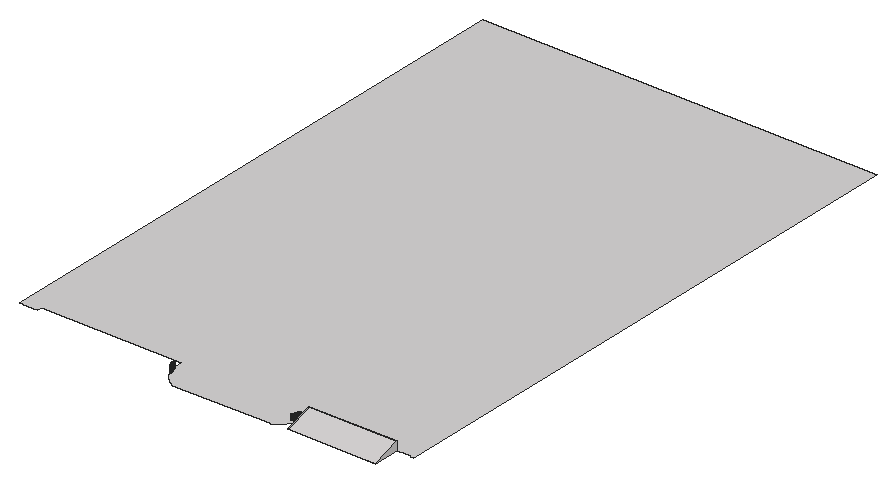
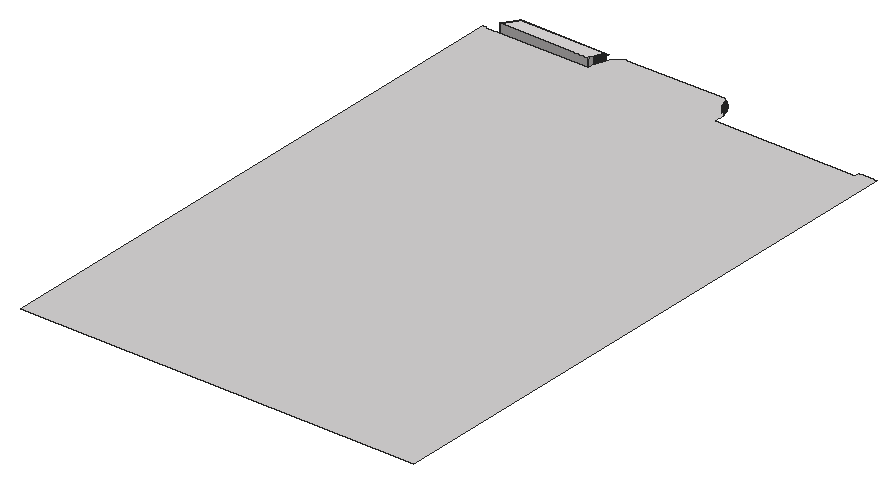
# SketchUp Ruby script. Lengths in inches.
U = 1.inch
M = Sketchup.active_model
def pt(a) = Geom::Point3d.new(a.map { |v| v * U })
def face(e, loops, mat)
  f = e.add_face(loops[0].map { |a| pt(a) })
  loops[1..].each { |l| e.add_face(l.map { |a| pt(a) }).erase! }
  f.material = f.back_material = mat if mat
  f
end
# faces: each face lists its corners as indices into pts; further lists are holes
def faces(e, pts, list, mat = nil) = list.each { |f| face(e, (f[0].is_a?(Array) ? f : [f]).map { |l| l.map { |i| pts[i] } }, mat) }
# xy, xz, yz: faces in a plane at the given z, y or x. An outline is a flat list of corners, or four numbers for a rectangle; further outlines are holes
def ring(l) = l.size == 4 ? [[l[0], l[1]], [l[2], l[1]], [l[2], l[3]], [l[0], l[3]]] : l.each_slice(2).to_a
def flat(e, list, mat, &to3) = list.each { |f| face(e, (f[0].is_a?(Array) ? f : [f]).map { |l| ring(l).map { |u, v| to3.(u, v) } }, mat) }
def xy(e, z, list, mat = nil) = flat(e, list, mat) { |x, y| [x, y, z] }
def xz(e, y, list, mat = nil) = flat(e, list, mat) { |x, z| [x, y, z] }
def yz(e, x, list, mat = nil) = flat(e, list, mat) { |y, z| [x, y, z] }
def lines(e, pts, list) = list.each { |a, b| e.add_line(pt(pts[a]), pt(pts[b])) }
# prism: a flat outline (further loops are holes) pulled along v
def prism(e, loops, v, mat = nil)
  f = face(e, loops, mat); d = Geom::Vector3d.new(v.map { |x| x * U })
  f.pushpull(f.normal.samedirection?(d) ? d.length : -d.length)
end
def box(e, o, s, mat = nil) = prism(e, [[o, [o[0] + s[0], o[1], o[2]], [o[0] + s[0], o[1] + s[1], o[2]], [o[0], o[1] + s[1], o[2]]]], [0, 0, s[2]], mat)
def at(x, y, z, deg = 0) = Geom::Transformation.translation(pt([x, y, z])) * Geom::Transformation.rotation(ORIGIN, Z_AXIS, deg.degrees)
def axes(o, x, y, z) = Geom::Transformation.new([*x, 0, *y, 0, *z, 0, *pt(o).to_a, 1])
def part(name) = M.definitions.add(name)
# library, detail: a bought-in or finely detailed component or shape, given as its bounding box
def library(name, o, s) = part(name).tap { |d| box(d.entities, o, s) }
def detail(e, o, s) = box(e.add_group.entities, o, s)
def put(e, d, t, mat = nil) = e.add_instance(d, t).tap { |i| i.material = mat if mat }
def group(e, t, mat = nil) = e.add_group.tap { |g| g.transformation = t; g.material = mat if mat }.entities
root = M.entities
M.materials.add("[Quartz Light Brown]").color = [215, 212, 212]
M.materials.add("[Stone Sandstone Ashlar Light]").color = [201, 199, 196]
xy(root,-12,[[240,0,239.65,0.16,239.29,0.32,238.59,0.66,238.25,0.83,237.9,1.01,237.56,1.19,237.21,1.375,236.53,1.75,236.2,1.95,235.86,2.14,235.2,2.54,234.21,3.17,232.93,4.05,232.62,4.28,232.3,4.51,231.99,4.74,231.6875,4.98,231.38,5.22,231.08,5.46,230.18,6.21,229.89,6.46,229.59,6.72,229.31,6.98,229.02,7.24,228.73,7.51,228.45,7.77,227.9,8.32,227.625,8.59,227.35,8.87,227.08,9.15,226.82,9.4375,226.56,9.72,226.04,10.3,225.78,10.6,225.53,10.89,225.28,11.19,225.04,11.49,224.79,11.79,224.55,12.1,224.32,12.41,224.08,12.72,223.62,13.34,223.4,13.66,223.17,13.98,222.95,14.3,222.53,14.95,222.32,15.28,222.11,15.6,221.91,15.9375,221.7,16.27,221.51,16.6,221.3125,16.94,221.12,17.28,220.94,17.62,220.75,17.96,220.57,18.31,220.39,18.65,219.88,19.7,219.72,20.05,219.55,20.4,219.4,20.76,219.24,21.12,219.09,21.47,218.95,21.83,218.8,22.2,218.52,22.92,218.39,23.29,218.26,23.65,218.14,24.02,218.01,24.39,217.89,24.76,217.67,25.5,217.45,26.25,217.25,27,217.07,27.76,216.98,28.13,216.82,28.89,216.74,29.28,216.6,30.04,216.54,30.42,216.48,30.81,216.42,31.19,216.36,31.58,216.31,31.96,216.27,32.35,216.23,32.73,216.1875,33.12,216.15,33.51,216.12,33.89,216.09,34.28,216.03,35.45,216.02,35.83,216,36.61,216,44,24,44,24,38,20,38,20,39,19,39,19,38,5,38,5,39,4,39,4,38,0,38,0,830,540,830,540,38,536,38,536,39,535,39,535,38,521,38,521,39,520,39,520,38,396,38,396,36,395.99,36,395.98,35.83,395.97,35.45,395.91,34.28,395.88,33.89,395.85,33.51,395.8125,33.12,395.77,32.73,395.73,32.35,395.69,31.96,395.64,31.58,395.58,31.19,395.52,30.81,395.46,30.42,395.4,30.04,395.26,29.28,395.18,28.89,395.02,28.13,394.93,27.76,394.75,27,394.55,26.25,394.33,25.5,394.11,24.76,393.99,24.39,393.86,24.02,393.74,23.65,393.61,23.29,393.48,22.92,393.2,22.2,393.05,21.83,392.91,21.47,392.76,21.12,392.6,20.76,392.45,20.4,392.28,20.05,392.12,19.7,391.61,18.65,391.43,18.31,391.25,17.96,391.06,17.62,390.88,17.28,390.6875,16.94,390.49,16.6,390.3,16.27,390.09,15.9375,389.89,15.6,389.68,15.28,389.47,14.95,389.05,14.3,388.83,13.98,388.6,13.66,388.38,13.34,387.92,12.72,387.68,12.41,387.45,12.1,387.21,11.79,386.96,11.49,386.72,11.19,386.47,10.89,386.22,10.6,385.96,10.3,385.44,9.72,385.18,9.4375,384.92,9.15,384.65,8.87,384.375,8.59,384.1,8.32,383.55,7.77,383.27,7.51,382.98,7.24,382.69,6.98,382.41,6.72,382.11,6.46,381.82,6.21,380.92,5.46,380.62,5.22,380.3125,4.98,380.01,4.74,379.7,4.51,379.38,4.28,379.07,4.05,377.79,3.17,376.8,2.54,376.14,2.14,375.8,1.95,375.47,1.75,374.79,1.375,374.44,1.19,374.1,1.01,373.75,0.83,373.41,0.66,372.71,0.32,372.35,0.16,372,0]],"[Quartz Light Brown]")
p = [[221.12,17.28,-3],[220.94,17.62,-3],[220.94,17.62,-12],[221.12,17.28,-12],[391.06,17.62,-3],[390.88,17.28,-3],
  [390.88,17.28,-12],[391.06,17.62,-12],[220.75,17.96,-3],[220.75,17.96,-12],[391.25,17.96,-3],[391.25,17.96,-12],
  [220.57,18.31,-3],[220.57,18.31,-12],[391.43,18.31,-3],[391.43,18.31,-12],[220.39,18.65,-3],[220.39,18.65,-12],
  [391.61,18.65,-3],[391.61,18.65,-12],[220.22,19,-3],[220.22,19,-12],[391.78,19,-3],[391.78,19,-12],
  [220.05,19.35,-3],[220.05,19.35,-12],[391.95,19.35,-3],[391.95,19.35,-12],[219.88,19.7,-3],[219.88,19.7,-12],
  [392.12,19.7,-3],[392.12,19.7,-12],[219.72,20.05,-3],[219.72,20.05,-12],[392.28,20.05,-3],[392.28,20.05,-12],
  [219.55,20.4,-3],[219.55,20.4,-12],[392.45,20.4,-3],[392.45,20.4,-12],[219.4,20.76,-3],[219.4,20.76,-12],
  [392.6,20.76,-3],[392.6,20.76,-12],[219.24,21.12,-3],[219.24,21.12,-12],[392.76,21.12,-3],[392.76,21.12,-12],
  [219.09,21.47,-3],[219.09,21.47,-12],[392.91,21.47,-3],[392.91,21.47,-12],[218.95,21.83,-3],[218.95,21.83,-12],
  [393.05,21.83,-3],[393.05,21.83,-12],[218.8,22.2,-3],[218.8,22.2,-12],[393.2,22.2,-3],[393.2,22.2,-12],
  [218.66,22.56,-3],[218.66,22.56,-12],[393.34,22.56,-3],[393.34,22.56,-12],[218.52,22.92,-3],[218.52,22.92,-12],
  [393.48,22.92,-3],[393.48,22.92,-12],[218.39,23.29,-3],[218.39,23.29,-12],[393.61,23.29,-3],[393.61,23.29,-12],
  [218.26,23.65,-3],[218.26,23.65,-12],[393.74,23.65,-3],[393.74,23.65,-12],[218.14,24.02,-3],[218.14,24.02,-12],
  [393.86,24.02,-3],[393.86,24.02,-12],[218.01,24.39,-3],[218.01,24.39,-12],[393.99,24.39,-3],[393.99,24.39,-12],
  [217.89,24.76,-3],[217.89,24.76,-12],[394.11,24.76,-3],[394.11,24.76,-12],[217.78,25.13,-3],[217.78,25.13,-12],
  [394.22,25.13,-3],[394.22,25.13,-12],[217.67,25.5,-3],[217.67,25.5,-12],[394.33,25.5,-3],[394.33,25.5,-12],
  [217.56,25.875,-3],[217.56,25.875,-12],[394.44,25.875,-3],[394.44,25.875,-12],[217.45,26.25,-3],[217.45,26.25,-12],
  [394.55,26.25,-3],[394.55,26.25,-12],[217.35,26.625,-3],[217.35,26.625,-12],[394.65,26.625,-3],[394.65,26.625,-12],
  [217.25,27,-3],[217.25,27,-12],[394.75,27,-3],[394.75,27,-12],[217.16,27.38,-3],[217.16,27.38,-12],
  [394.84,27.38,-3],[394.84,27.38,-12],[217.07,27.76,-3],[217.07,27.76,-12],[394.93,27.76,-3],[394.93,27.76,-12],
  [216.98,28.13,-3],[216.98,28.13,-12],[395.02,28.13,-3],[395.02,28.13,-12],[224.47,17.5,-3],[224.66,17.1875,-3],
  [224.66,17.1875,-10],[224.47,17.5,-10],[387.34,17.1875,-3],[387.53,17.5,-3],[387.53,17.5,-10],[387.34,17.1875,-10],
  [224.28,17.8,-3],[224.28,17.8,-10],[387.72,17.8,-3],[387.72,17.8,-10],[224.1,18.11,-3],[224.1,18.11,-10],
  [387.9,18.11,-3],[387.9,18.11,-10],[223.92,18.43,-3],[223.92,18.43,-10],[388.08,18.43,-3],[388.08,18.43,-10],
  [223.74,18.74,-3],[223.74,18.74,-10],[388.26,18.74,-3],[388.26,18.74,-10],[223.57,19.05,-3],[223.57,19.05,-10],
  [388.43,19.05,-3],[388.43,19.05,-10],[223.4,19.37,-3],[223.4,19.37,-10],[388.6,19.37,-3],[388.6,19.37,-10],
  [223.23,19.69,-3],[223.23,19.69,-10],[388.77,19.69,-3],[388.77,19.69,-10],[223.07,20.01,-3],[223.07,20.01,-10],
  [388.93,20.01,-3],[388.93,20.01,-10],[222.91,20.33,-3],[222.91,20.33,-10],[389.09,20.33,-3],[389.09,20.33,-10],
  [222.75,20.65,-3],[222.75,20.65,-10],[389.25,20.65,-3],[389.25,20.65,-10],[222.59,20.98,-3],[222.59,20.98,-10],
  [389.41,20.98,-3],[389.41,20.98,-10],[222.44,21.31,-3],[222.44,21.31,-10],[389.56,21.31,-3],[389.56,21.31,-10],
  [222.29,21.63,-3],[222.29,21.63,-10],[389.71,21.63,-3],[389.71,21.63,-10],[222.15,21.96,-3],[222.15,21.96,-10],
  [389.85,21.96,-3],[389.85,21.96,-10],[222,22.29,-3],[222,22.29,-10],[390,22.29,-3],[390,22.29,-10],
  [221.86,22.625,-3],[221.86,22.625,-10],[390.14,22.625,-3],[390.14,22.625,-10],[221.73,22.96,-3],[221.73,22.96,-10],
  [390.27,22.96,-3],[390.27,22.96,-10],[221.59,23.29,-3],[221.59,23.29,-10],[390.41,23.29,-3],[390.41,23.29,-10],
  [221.46,23.625,-3],[221.46,23.625,-10],[390.54,23.625,-3],[390.54,23.625,-10],[221.34,23.96,-3],[221.34,23.96,-10],
  [390.66,23.96,-3],[390.66,23.96,-10],[221.21,24.3,-3],[221.21,24.3,-10],[390.79,24.3,-3],[390.79,24.3,-10],
  [221.09,24.64,-3],[221.09,24.64,-10],[390.91,24.64,-3],[390.91,24.64,-10],[220.98,24.98,-3],[220.98,24.98,-10],
  [391.02,24.98,-3],[391.02,24.98,-10],[220.86,25.32,-3],[220.86,25.32,-10],[391.14,25.32,-3],[391.14,25.32,-10],
  [220.75,25.67,-3],[220.75,25.67,-10],[391.25,25.67,-3],[391.25,25.67,-10],[220.65,26.01,-3],[220.65,26.01,-10],
  [391.35,26.01,-3],[391.35,26.01,-10],[220.54,26.35,-3],[220.54,26.35,-10],[391.46,26.35,-3],[391.46,26.35,-10],
  [220.44,26.7,-3],[220.44,26.7,-10],[391.56,26.7,-3],[391.56,26.7,-10],[220.34,27.05,-3],[220.34,27.05,-10],
  [391.66,27.05,-3],[391.66,27.05,-10],[220.25,27.39,-3],[220.25,27.39,-10],[391.75,27.39,-3],[391.75,27.39,-10],
  [220.16,27.74,-3],[220.16,27.74,-10],[391.84,27.74,-3],[391.84,27.74,-10],[220.07,28.09,-3],[220.07,28.09,-10],
  [391.93,28.09,-3],[391.93,28.09,-10],[219.99,28.44,-3],[219.99,28.44,-10],[392.01,28.44,-3],[392.01,28.44,-10]]
faces(root,p,[[0,1,2,3],[4,5,6,7],[1,8,9,2],[10,4,7,11],[8,12,13,9],[14,10,11,15],[12,16,17,13],[18,14,15,19],
  [16,20,21,17],[22,18,19,23],[20,24,25,21],[26,22,23,27],[24,28,29,25],[30,26,27,31],[28,32,33,29],[34,30,31,35],
  [32,36,37,33],[38,34,35,39],[36,40,41,37],[42,38,39,43],[40,44,45,41],[46,42,43,47],[44,48,49,45],[50,46,47,51],
  [48,52,53,49],[54,50,51,55],[52,56,57,53],[58,54,55,59],[56,60,61,57],[62,58,59,63],[60,64,65,61],[66,62,63,67],
  [64,68,69,65],[70,66,67,71],[68,72,73,69],[74,70,71,75],[72,76,77,73],[78,74,75,79],[76,80,81,77],[82,78,79,83],
  [80,84,85,81],[86,82,83,87],[84,88,89,85],[90,86,87,91],[88,92,93,89],[94,90,91,95],[92,96,97,93],[98,94,95,99],
  [96,100,101,97],[102,98,99,103],[100,104,105,101],[106,102,103,107],[104,108,109,105],[110,106,107,111],[108,112,113,109],[114,110,111,115],
  [112,116,117,113],[118,114,115,119],[116,120,121,117],[122,118,119,123],[124,125,126,127],[128,129,130,131],[132,124,127,133],[129,134,135,130],
  [136,132,133,137],[134,138,139,135],[140,136,137,141],[138,142,143,139],[144,140,141,145],[142,146,147,143],[148,144,145,149],[146,150,151,147],
  [152,148,149,153],[150,154,155,151],[156,152,153,157],[154,158,159,155],[160,156,157,161],[158,162,163,159],[164,160,161,165],[162,166,167,163],
  [168,164,165,169],[166,170,171,167],[172,168,169,173],[170,174,175,171],[176,172,173,177],[174,178,179,175],[180,176,177,181],[178,182,183,179],
  [184,180,181,185],[182,186,187,183],[188,184,185,189],[186,190,191,187],[192,188,189,193],[190,194,195,191],[196,192,193,197],[194,198,199,195],
  [200,196,197,201],[198,202,203,199],[204,200,201,205],[202,206,207,203],[208,204,205,209],[206,210,211,207],[212,208,209,213],[210,214,215,211],
  [216,212,213,217],[214,218,219,215],[220,216,217,221],[218,222,223,219],[224,220,221,225],[222,226,227,223],[228,224,225,229],[226,230,231,227],
  [232,228,229,233],[230,234,235,231],[236,232,233,237],[234,238,239,235],[240,236,237,241],[238,242,243,239],[244,240,241,245],[242,246,247,243],
  [248,244,245,249],[246,250,251,247],[252,248,249,253],[250,254,255,251],[256,252,253,257],[254,258,259,255],[260,256,257,261],[258,262,263,259]],"[Stone Sandstone Ashlar Light]")
g1 = group(root,at(396,2,-12),"[Quartz Light Brown]")
xy(g1,0,[[0,0,120,36]])
xz(g1,36,[[0,0,120,12]])
yz(g1,0,[[0,0,34,11.33,34,0],[34,0,34,11.33,36,12,36,0]])
yz(g1,120,[[0,0,36,0,36,12]])
p = [[0,0,0],[120,0,0],[120,36,12],[0,36,12],[0,34,11.33]]
faces(g1,p,[[0,1,2,3,4]])
